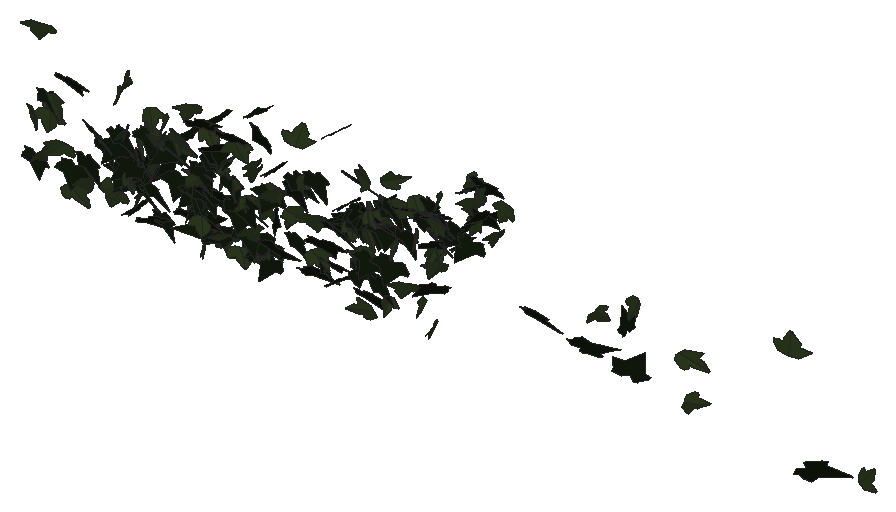
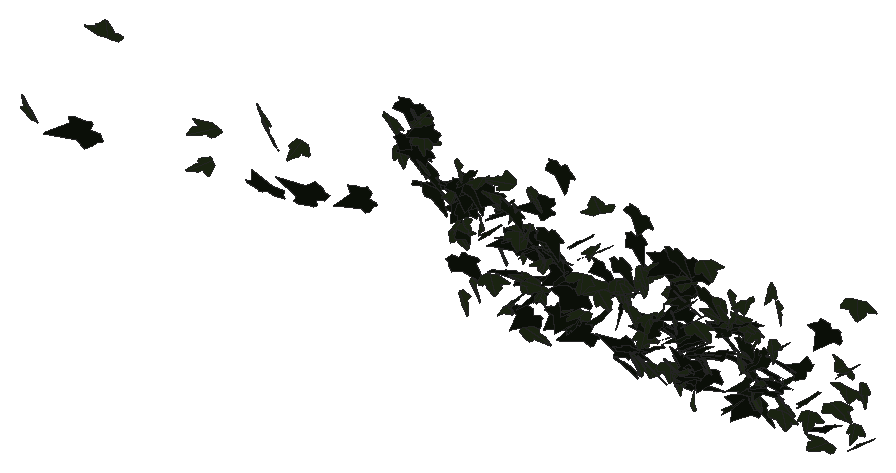
# SketchUp Ruby script. Lengths in millimetres.
U = 1.mm
M = Sketchup.active_model
def pt(a) = Geom::Point3d.new(a.map { |v| v * U })
def face(e, loops, mat)
  f = e.add_face(loops[0].map { |a| pt(a) })
  loops[1..].each { |l| e.add_face(l.map { |a| pt(a) }).erase! }
  f.material = f.back_material = mat if mat
  f
end
# faces: each face lists its corners as indices into pts; further lists are holes
def faces(e, pts, list, mat = nil) = list.each { |f| face(e, (f[0].is_a?(Array) ? f : [f]).map { |l| l.map { |i| pts[i] } }, mat) }
# xy, xz, yz: faces in a plane at the given z, y or x. An outline is a flat list of corners, or four numbers for a rectangle; further outlines are holes
def ring(l) = l.size == 4 ? [[l[0], l[1]], [l[2], l[1]], [l[2], l[3]], [l[0], l[3]]] : l.each_slice(2).to_a
def flat(e, list, mat, &to3) = list.each { |f| face(e, (f[0].is_a?(Array) ? f : [f]).map { |l| ring(l).map { |u, v| to3.(u, v) } }, mat) }
def xy(e, z, list, mat = nil) = flat(e, list, mat) { |x, y| [x, y, z] }
def xz(e, y, list, mat = nil) = flat(e, list, mat) { |x, z| [x, y, z] }
def yz(e, x, list, mat = nil) = flat(e, list, mat) { |y, z| [x, y, z] }
def lines(e, pts, list) = list.each { |a, b| e.add_line(pt(pts[a]), pt(pts[b])) }
# prism: a flat outline (further loops are holes) pulled along v
def prism(e, loops, v, mat = nil)
  f = face(e, loops, mat); d = Geom::Vector3d.new(v.map { |x| x * U })
  f.pushpull(f.normal.samedirection?(d) ? d.length : -d.length)
end
def box(e, o, s, mat = nil) = prism(e, [[o, [o[0] + s[0], o[1], o[2]], [o[0] + s[0], o[1] + s[1], o[2]], [o[0], o[1] + s[1], o[2]]]], [0, 0, s[2]], mat)
def at(x, y, z, deg = 0) = Geom::Transformation.translation(pt([x, y, z])) * Geom::Transformation.rotation(ORIGIN, Z_AXIS, deg.degrees)
def axes(o, x, y, z) = Geom::Transformation.new([*x, 0, *y, 0, *z, 0, *pt(o).to_a, 1])
def part(name) = M.definitions.add(name)
# library, detail: a bought-in or finely detailed component or shape, given as its bounding box
def library(name, o, s) = part(name).tap { |d| box(d.entities, o, s) }
def detail(e, o, s) = box(e.add_group.entities, o, s)
def put(e, d, t, mat = nil) = e.add_instance(d, t).tap { |i| i.material = mat if mat }
def group(e, t, mat = nil) = e.add_group.tap { |g| g.transformation = t; g.material = mat if mat }.entities
root = M.entities
M.materials.add("efeu1").color = [18, 25, 13]
M.materials.add("efeu2").color = [43, 57, 29]
c1 = part("ivyleaf_9")
p = [[39.1,54.8,31.7],[34.5,51.8,30.2],[-5.3,25.2,17.3],[-17.9,28.3,20.9],[-21.6,21.7,17],[-20.2,4.3,5.3],
  [-22.9,-0.3,2.5],[-17.1,-4,-0.6],[-2,-2.1,-1.2],[-0.7,-15.4,-10.1],[16.6,-22.3,-16.7],[21.1,-15.1,-12.5],
  [32.7,-10.7,-11],[46.1,-1.8,-6.6],[30.8,11.2,3.8]]
faces(c1.entities,p,[[0,1,2,3,4,5,6,7,8,9,10,11,12,13,14]],"efeu1")
c2 = part("ivyleaf_10")
p = [[0,12.8,-0.8],[-1.5,51.3,-10.9],[-4.9,51,-11.6],[-13.6,26.5,-7.3],[-13.2,15.9,-4.6],[-21.1,19.3,-7.2],
  [-29.5,16.3,-8.3],[-29.2,8.3,-6.2],[-19.7,-9.8,0.5],[-7.6,-13,4],[1,-12.2,5.8],[-0.4,51.1,-11.1],
  [-1.5,51.1,-10.9],[1,-12.4,5.9],[16.9,-12.4,3.5],[35.1,9.1,-5.1],[35,12.9,-6.1],[20.5,16.4,-4.9],
  [15.8,15,-3.8],[15.3,27.6,-7.1],[12.8,31.3,-7.8]]
faces(c2.entities,p,[[0,1,2,3,4,5,6,7,8,9,10],[11,12,0,13,14,15,16,17,18,19,20]],"efeu2")
put(root,c1,axes([3669.9,850.2,2672.9],[-0.17416,-1.02117,0.24086],[0.05118,-0.24398,-1.02417],[1.99617,-0.08284,0.04727]))
put(root,c2,axes([3698,804.6,2852.7],[1.08646,-0.66517,-0.85461],[-0.32174,0.8995,-0.81303],[2.03584,0.49713,0.32759]))
put(root,c2,axes([3702,829.9,3173.5],[-1.91435,-0.41148,0.06163],[-0.09912,-0.03545,-1.08669],[0.78563,-1.00712,0.01307]))
put(root,c2,axes([3711.1,828.5,2709.7],[-0.45389,-0.87585,-0.50942],[0.33295,0.47989,-0.90698],[1.89941,-0.29342,0.03725]))
put(root,c2,axes([3731.6,839.8,2852.3],[2.11144,-0.10197,0.14703],[0.2783,-0.01543,-1.11409],[0.19625,1.11901,-0.00197]))
put(root,c1,axes([3727.3,840.6,2921.2],[0.28219,-1.05732,0.05783],[0.00332,-0.05815,-1.06765],[2.0153,0.14814,-0.00634]))
put(root,c2,axes([3795,827.5,2761.8],[1.50681,0.45752,-0.55032],[-1.16763,0.01134,-0.87321],[-0.70132,0.96413,0.27142]))
put(root,c2,axes([3752.5,827.9,2920.7],[1.49914,-0.25929,0.7659],[1.37117,-0.26042,-0.82911],[0.69872,1.06736,-0.01623]))
put(root,c1,axes([3825.1,852.5,2684.6],[-0.7651,-0.96985,0.04167],[0.03243,-0.05214,-1.04926],[1.84724,-0.40078,0.03568]))
put(root,c1,axes([3826.2,813.7,3026.5],[1.96393,0.14353,-0.33162],[-0.64116,0.01922,-1.03998],[-0.24874,1.08372,0.06236]))
put(root,c2,axes([3834,833.2,2613.2],[1.53063,0.2367,0.68994],[1.21346,0.2707,-0.83609],[-0.67428,1.02447,0.06152]))
put(root,c2,axes([3909.3,817.4,2683.3],[-0.93066,-0.9112,-0.30006],[0.28233,0.26092,-1.03409],[1.80384,-0.51096,0.00704]))
put(root,c1,axes([3896.6,827.7,2751.1],[0.49702,-1.06639,0.03219],[0.01281,-0.03149,-1.0979],[2.03043,0.26123,-0.00095]))
put(root,c1,axes([3907.3,841.6,2857.7],[0.88542,-0.86766,0.51882],[0.44377,-0.46363,-0.98444],[1.87216,0.52025,-0.01202]))
put(root,c1,axes([3950,852.6,2817.6],[0.30365,-1.01846,0.19997],[-0.01159,-0.20323,-1.03023],[1.97532,0.15537,-0.03678]))
put(root,c2,axes([4005.9,837.7,2660.8],[-1.9519,0.1001,0.18014],[-0.38341,-0.29426,-0.98343],[-0.08266,-0.99885,0.30777]))
put(root,c2,axes([3987.3,824.9,2671.6],[1.19853,-0.51065,-0.74179],[1.10381,-0.46249,0.81075],[-1.31119,-0.85611,0.00447]))
put(root,c1,axes([4031,830.3,2846.2],[-1.86698,-0.11127,-0.32265],[0.64458,-0.19605,-0.96211],[0.08025,-1.01389,0.22145]))
put(root,c2,axes([4035,820.4,3043.2],[0.50605,-1.0177,-0.32096],[-0.02478,0.32766,-1.04972],[2.03079,0.2576,0.06717]))
put(root,c2,axes([4048.1,832.6,2902.6],[-0.09626,-1.0225,-0.34592],[0.03967,0.34531,-1.02375],[2.05399,-0.05459,0.00356]))
put(root,c1,axes([4022.3,827.8,2895.6],[0.75234,-0.92591,-0.37005],[-0.05692,0.38688,-0.99997],[1.89686,0.37885,0.11677]))
put(root,c1,axes([4061.6,835.9,2765.1],[-1.7575,-0.44266,-0.19578],[0.41975,-0.00942,-1.01897],[0.82001,-0.94392,0.10198]))
put(root,c2,axes([4062.8,818.3,3098.6],[-0.02086,-0.65902,-0.96601],[0.22835,0.96032,-0.6565],[2.21385,-0.10526,0.05862]))
put(root,c1,axes([4087.1,854.6,2731.2],[-1.76538,-0.435,0.22936],[-0.26059,-0.24184,-1.01243],[0.89891,-0.92441,0.15694]))
put(root,c1,axes([4097.6,826.9,2795],[-1.98395,-0.01938,-0.09874],[0.1908,-0.11215,-1.03642],[0.01638,-1.04107,0.11349]))
put(root,c2,axes([4081.3,814.1,2754.9],[0.35376,1.01356,0.0054],[0.0015,0.00535,-1.03046],[-1.92904,0.18588,0.00019]))
put(root,c1,axes([4083.3,825.5,2841.4],[1.72957,-0.34909,-0.4459],[-0.63884,0.34699,-0.95576],[0.86803,0.95094,0.18506]))
put(root,c2,axes([4108.4,846.9,2692],[0.40459,-0.97969,0.34164],[0.16515,-0.33073,-1.00239],[1.96775,0.22919,0.01388]))
put(root,c1,axes([4129.1,811.5,2661.6],[-0.80767,0.97747,-0.16961],[0.0991,-0.16227,-1.06549],[-1.88551,-0.42723,0.01665]))
put(root,c1,axes([4094.3,836.4,2721.9],[1.22771,-0.84105,0.05564],[0.06813,-0.04266,-1.05994],[1.60273,0.64606,0.00244]))
put(root,c1,axes([4115.8,829.1,2836.4],[1.34795,-0.38353,-0.67717],[-0.93971,0.48628,-0.79184],[1.14486,0.85071,0.14734]))
put(root,c2,axes([4120.2,817.8,2896.3],[-0.42117,0.99873,-0.22509],[0.02091,-0.22796,-1.02226],[-1.94835,-0.21834,0.03769]))
put(root,c1,axes([4153,827.4,2784.3],[-1.32671,0.647,-0.42557],[0.57818,-0.29823,-0.95102],[-1.35574,-0.76034,0.01088]))
put(root,c2,axes([4134.7,824.8,2921.7],[-1.59669,0.59742,-0.21327],[0.26377,-0.17244,-1.02824],[-1.17811,-0.84829,0.05882]))
put(root,c2,axes([4182.9,824.6,2936.6],[-0.69387,0.14567,0.98024],[-1.87868,-0.14573,-0.34549],[0.16677,-1.03564,0.18649]))
put(root,c2,axes([4156.7,846.4,2808.4],[0.14279,-1.03808,0.12585],[0.06015,-0.12387,-1.04054],[1.98922,0.07826,0.02243]))
put(root,c1,axes([4178.1,818.3,2858.8],[-0.83606,0.95911,-0.06774],[0.07245,-0.05707,-1.05487],[-1.82849,-0.4408,-0.01082]))
put(root,c1,axes([4140.3,843.7,2730.1],[1.07875,-0.86114,-0.13041],[-0.03014,0.14537,-1.02881],[1.65733,0.56316,0.06617]))
put(root,c1,axes([4176.4,845.9,2812.9],[-1.85704,-0.34148,-0.20869],[0.41497,0.00754,-1.03181],[0.63868,-0.99779,0.06362]))
put(root,c2,axes([4164.5,823.6,3016.1],[0.56951,1.09198,-0.17073],[-0.11915,-0.15984,-1.1321],[-2.10014,0.30519,0.01793]))
put(root,c2,axes([4168.5,843.2,2811.6],[0.15033,-0.95431,0.43372],[0.34481,-0.41598,-0.94826],[1.965,0.146,0.13322]))
put(root,c1,axes([4172.3,830.6,2932.7],[-0.9679,-0.94321,-0.09432],[0.05731,0.0909,-1.07145],[1.80315,-0.50918,-0.01657]))
put(root,c1,axes([4167.8,806.6,2633.6],[1.50685,0.67685,0.12793],[0.18914,0.08063,-1.04162],[-1.29727,0.79795,-0.00327]))
put(root,c2,axes([4216.9,814,2927.6],[0.00117,0.13162,1.05151],[-0.66028,0.99359,-0.12416],[-1.9057,-0.34418,0.04367]))
put(root,c1,axes([4191.7,850.7,2632.8],[0.43653,-1.0033,0.0634],[-0.00129,-0.06518,-1.02908],[1.9133,0.22886,-0.01516]))
put(root,c2,axes([4227,822.5,3010.4],[0.64338,-1.0447,-0.00092],[0.01246,0.00309,-1.09801],[1.98823,0.33804,0.00718]))
put(root,c1,axes([4245.4,831.4,2865.2],[-1.54309,0.45568,-0.52869],[0.81465,-0.31545,-0.92833],[-1.04923,-0.91508,0.05675]))
put(root,c1,axes([4257.9,833.9,2903.9],[-1.79694,-0.47383,0.23394],[-0.4188,-0.08294,-1.05612],[0.91437,-0.96918,-0.02399]))
put(root,c1,axes([4215.5,842.9,2901.1],[0.74292,-0.86605,0.48781],[0.78845,-0.33463,-0.92562],[1.7196,0.52759,0.21365]))
put(root,c1,axes([4269.6,847.4,2801.7],[-1.03337,-0.90726,0.00395],[-0.00347,-0.00351,-1.05732],[1.72671,-0.54297,0.00024]))
put(root,c2,axes([4278.6,820.6,2970.8],[-1.64011,0.59298,0.20748],[-0.33821,0.10774,-1.04601],[-1.14683,-0.87982,0.01175]))
put(root,c2,axes([4244.5,840.7,2927.8],[0.12335,0.0127,1.18772],[2.24987,-0.11645,-0.06326],[0.22,1.18378,-0.01897]))
put(root,c1,axes([4334.6,831.2,2996.4],[-0.87454,0.96714,0.04112],[-0.04025,0.03548,-1.07075],[-1.84189,-0.45998,0.00387]))
put(root,c2,axes([4330.7,823.2,3093.5],[-1.14244,-0.87702,0.25844],[-0.11213,-0.27142,-1.0579],[1.7365,-0.59452,0.10172]))
put(root,c2,axes([4318.2,835.9,2745.1],[1.00135,-0.83541,0.33377],[0.48748,-0.23155,-0.98332],[1.64129,0.57846,0.08842]))
put(root,c1,axes([4337.5,853.1,2770.8],[-1.42849,-0.65112,0.33645],[-0.2605,-0.34857,-0.97993],[1.37032,-0.74502,0.16444]))
put(root,c1,axes([4321.9,822,2706],[1.55032,0.65168,-0.14431],[-0.2017,-0.09852,-1.04313],[-1.2542,0.82138,-0.01063]))
put(root,c2,axes([4373.2,824,2851.9],[-1.51746,-0.32726,0.62113],[-0.85896,-0.48102,-0.83279],[1.0235,-0.8889,0.22198]))
put(root,c1,axes([4365.1,828.3,2752.5],[-1.41251,0.35638,-0.65274],[1.00684,-0.39515,-0.81725],[-0.99479,-0.90596,0.09968]))
put(root,c1,axes([4354.6,844.3,2777.7],[-0.62927,-0.97685,0.19643],[-0.18843,-0.17372,-1.03061],[1.88697,-0.34311,-0.03741]))
put(root,c1,axes([4399.2,848.8,2648.1],[-1.46775,-0.11484,0.84238],[-1.57813,-0.14946,-0.77951],[0.35718,-1.13226,0.01746]))
put(root,c1,axes([4365.4,843.1,2783.7],[-0.4246,-1.0258,0.17771],[-0.02906,-0.1785,-1.04953],[1.98117,-0.22246,0.02269]))
put(root,c2,axes([4369.5,829.2,2689.7],[1.29866,0.80377,-0.07318],[-0.10086,-0.05101,-1.05432],[-1.53274,0.68437,0.00737]))
put(root,c2,axes([4362.5,848.8,2586.1],[0.1001,-0.06848,1.13998],[1.21539,-0.94434,-0.08619],[1.80196,0.64075,-0.00519]))
put(root,c1,axes([4365.9,832.2,2880.5],[0.18721,-1.07427,-0.09221],[-0.00741,0.09224,-1.07876],[2.05206,0.09834,0.00451]))
put(root,c1,axes([4363.5,808,3058.7],[1.9174,0.44244,0.15073],[0.26893,0.05309,-1.1003],[-0.84796,1.01729,-0.00813]))
put(root,c1,axes([4352.4,850.4,2685.7],[0.48432,-0.52196,1.01173],[0.95764,-0.87837,-0.57972],[1.94355,0.56287,0.03353]))
put(root,c1,axes([4374.1,843.6,2794.6],[-0.04482,-1.03029,-0.27005],[-0.00316,0.27015,-1.03053],[2.02708,-0.02236,-0.00758]))
put(root,c1,axes([4363.2,841.3,2694.5],[-0.10504,-0.06408,1.06097],[1.40093,-0.76871,-0.00814],[1.45931,0.73335,0.08418]))
put(root,c2,axes([4395.8,832.6,3021.4],[1.09062,0.89184,0.18458],[0.16171,0.16478,-1.05994],[-1.72577,0.57905,0.01733]))
put(root,c1,axes([4410.4,813.4,2817.5],[1.73249,0.44583,-0.40687],[-0.66916,-0.20676,-1.01321],[-0.9337,0.97542,-0.0288]))
put(root,c1,axes([4397.8,834.9,2925.5],[0.84187,-0.90867,-0.3788],[0.00024,0.41533,-0.99616],[1.87363,0.40823,0.17033]))
put(root,c1,axes([4396.3,830.2,2946],[1.17813,-0.89247,-0.02327],[0.1527,0.08382,-1.08017],[1.69225,0.61377,0.11367]))
put(root,c1,axes([4402.1,829.4,2906.2],[2.01072,-0.2578,-0.00147],[0.00427,0.01542,-1.08738],[0.49064,1.05638,0.01551]))
put(root,c1,axes([4453,828.8,3098.3],[-0.66563,1.02892,-0.0112],[-0.04779,-0.02036,-1.08631],[-1.95777,-0.34933,0.03033]))
put(root,c1,axes([4406.2,824.5,2809],[1.24895,-0.76037,-0.3642],[-0.11255,0.41887,-0.98107],[1.60062,0.62276,0.2152]))
put(root,c1,axes([4422.8,804.5,2987.1],[1.21972,0.75897,0.40754],[0.44216,0.33686,-0.99267],[-1.5788,0.68069,0.03685]))
put(root,c1,axes([4463.1,824.9,2949.7],[-1.81031,0.53547,0.04189],[-0.07388,0.01643,-1.09155],[-1.01955,-0.95197,0.00472]))
put(root,c2,axes([4442.9,835.3,2646.9],[1.41868,-0.61204,-0.39838],[-0.23898,0.45337,-0.93147],[1.36917,0.71331,0.25021]))
put(root,c2,axes([4453,838,2870.4],[0.75404,-0.96529,-0.257],[-0.01266,0.27392,-1.0391],[1.90109,0.38469,0.09501]))
put(root,c1,axes([4484.3,820.7,2674.3],[-1.51842,0.64432,0.02333],[-0.10656,-0.03226,-1.02374],[-1.22244,-0.79751,0.06026]))
put(root,c2,axes([4477.7,821.8,2668.1],[-1.39467,-0.71537,-0.04037],[0.07193,0.01907,-1.02401],[1.36177,-0.73367,0.01274]))
put(root,c2,axes([4475.6,800.2,2930.5],[0.24157,-0.46512,1.05499],[-0.33937,1.04067,0.48026],[-2.16793,-0.21474,0.04237]))
put(root,c1,axes([4477,843.6,2871.7],[0.28825,-1.05206,0.06443],[0.0115,-0.06422,-1.0629],[2.006,0.15154,-0.00316]))
put(root,c1,axes([4480,815.2,3048.2],[2.06916,0.15846,-0.03375],[-0.07278,0.02847,-1.09817],[-0.29963,1.08735,0.03367]))
put(root,c2,axes([4506,827.9,2867.4],[-0.17968,0.97241,-0.40538],[-0.08339,-0.41028,-0.97395],[-2.00333,-0.07014,0.0769]))
put(root,c1,axes([4514.1,847.5,2758],[-0.60949,-0.94857,0.31634],[0.02002,-0.33535,-0.99491],[1.90296,-0.30029,0.11179]))
put(root,c2,axes([4519.8,822.6,3017.8],[-1.33014,-0.79219,-0.30752],[0.84674,-0.00187,-1.0063],[1.37794,-0.76356,0.32152]))
put(root,c2,axes([4545.6,838.2,2805.5],[-0.33284,-1.04729,0.05785],[0.37063,-0.09005,-1.0415],[1.96154,-0.16069,0.20661]))
put(root,c1,axes([4517.2,843.2,2801.3],[1.40006,-0.65,0.38792],[0.53049,-0.27032,-0.98152],[1.33941,0.78649,-0.01675]))
put(root,c1,axes([4528.8,823.8,2817.6],[-0.8672,-0.41074,-0.91799],[1.55562,0.43592,-0.60076],[1.11515,-0.92752,0.12417]))
put(root,c2,axes([4539.3,816.2,2640.4],[1.69923,0.43868,0.24577],[0.44332,0.08302,-0.9944],[-0.84812,0.92231,-0.02738]))
put(root,c1,axes([4582.6,828.7,2653],[-1.60207,0.56961,-0.05662],[0.09258,-0.02914,-1.01639],[-1.08549,-0.84318,-0.00312]))
put(root,c2,axes([4555.4,830.1,2827.2],[0.55785,1.02348,0.03769],[-0.11655,0.05665,-1.06202],[-1.94572,0.29004,0.07442]))
put(root,c1,axes([4557.1,832.1,2710.3],[-0.34319,-1.0131,-0.20221],[0.13937,0.19222,-1.02834],[1.96123,-0.19094,0.03769]))
put(root,c2,axes([4593.3,831,2952.4],[-0.33928,-1.06893,-0.03979],[-0.0385,0.0437,-1.08336],[2.03544,-0.17735,-0.02713]))
put(root,c2,axes([4593.8,825.1,2981],[-0.30344,-1.08106,0.02862],[0.00559,-0.02937,-1.09273],[2.05819,-0.1593,0.00719]))
put(root,c2,axes([4590.9,813.9,2737.8],[-0.91247,-0.90072,-0.37557],[0.38233,0.31839,-1.02004],[1.81752,-0.51917,0.02602]))
put(root,c1,axes([4619.9,822.4,3092.9],[0.87127,0.08634,-1.10755],[-2.10184,0.16518,-0.4436],[0.22912,1.187,0.14229]))
put(root,c1,axes([4607.5,811.1,3174.4],[0.56002,0.92645,0.52974],[-0.05912,0.55671,-0.95636],[-2.03025,0.23934,0.17397]))
put(root,c2,axes([4600.6,844.3,2657.3],[1.43932,-0.72269,0.01223],[-0.00551,-0.02073,-1.04591],[1.37561,0.75608,-0.01699]))
put(root,c2,axes([4612.2,843.2,2665.1],[1.54057,-0.66459,0.01205],[0.01534,-0.00917,-1.04734],[1.26497,0.8095,-0.00197]))
put(root,c1,axes([4643,850.9,2687.6],[-1.7581,-0.37392,0.24336],[-0.43404,-0.08518,-0.99654],[0.72977,-0.95147,-0.00642]))
put(root,c2,axes([4633,830.6,2829],[1.63471,-0.58825,-0.24217],[-0.17832,0.28548,-1.02575],[1.19752,0.84552,0.17785]))
put(root,c1,axes([4651.9,844.5,2628.3],[-1.77465,0.00042,-0.43465],[0.82072,-0.12795,-0.92524],[-0.1036,-1.0208,0.11579]))
put(root,c1,axes([4654.7,839.1,2879],[-1.18018,-0.82302,0.29027],[0.02945,-0.3664,-1.00581],[1.66067,-0.57839,0.22412]))
put(root,c1,axes([4676.9,833.5,2985.3],[-0.63203,1.01356,-0.1565],[0.05172,-0.15574,-1.06634],[-1.95117,-0.33244,0.02243]))
put(root,c2,axes([4666,832.4,2900.2],[1.53874,-0.67201,-0.18203],[-0.22898,0.1399,-1.05088],[1.30512,0.81685,0.03024]))
put(root,c2,axes([4667.7,818.6,2901.9],[-0.74413,-0.992,-0.26862],[0.18649,0.25011,-1.06627],[1.94706,-0.40308,-0.00053]))
put(root,c1,axes([4637.9,840.1,2674.4],[0.69436,-0.29991,0.91578],[1.4261,-0.52741,-0.47124],[1.15316,0.83283,0.03135]))
put(root,c1,axes([4689.9,806,2817.6],[0.48459,-0.22787,-1.11533],[-1.61743,0.72234,-0.34159],[1.44146,0.88713,-0.00834]))
put(root,c2,axes([4688.9,827.8,2900.2],[-0.76854,-0.99757,-0.03403],[-0.00695,0.03818,-1.07606],[1.89967,-0.40344,-0.0177]))
put(root,c2,axes([4749.6,836.6,2838.9],[-0.55176,-0.98191,0.31894],[-0.08655,-0.31881,-1.02284],[1.96297,-0.29006,0.04455]))
put(root,c1,axes([4737.2,837.7,2942.1],[-0.51716,-0.01761,-1.03792],[1.97531,0.01554,-0.27199],[0.03711,-1.07279,0.01309]))
put(root,c1,axes([4747.5,831.3,2757.9],[0.80289,-0.94909,-0.08441],[-0.0612,0.07808,-1.03862],[1.8124,0.42308,0.00232]))
put(root,c2,axes([4749.5,813,2855.6],[0.63511,0.3441,0.95667],[0.90244,0.838,-0.46681],[-1.7116,0.56952,0.10886]))
put(root,c2,axes([4776.1,809.2,3132.3],[1.40816,0.84599,-0.48301],[0.62082,0.35637,1.12384],[1.747,-0.80854,-0.01004]))
put(root,c1,axes([4764.8,816.8,2991.6],[0.76785,-0.89232,-0.45673],[0.05161,0.50187,-0.95656],[1.9071,0.34569,0.20978]))
put(root,c2,axes([4795.6,816.3,2990.5],[0.28172,1.07471,0.00521],[-0.01094,0.00605,-1.08483],[-2.04538,0.14799,0.00652]))
put(root,c2,axes([4841.7,822.5,2865.9],[-1.84788,-0.47407,-0.06035],[0.09767,0.03245,-1.08047],[0.90427,-0.97227,-0.00663]))
put(root,c1,axes([4818.6,815.9,2670.4],[1.8857,0.19349,0.34196],[0.63533,0.07469,-1.00948],[-0.39437,1.04549,0.00883]))
put(root,c1,axes([4833.7,831.3,3011.3],[0.21764,-1.05858,-0.20086],[-0.06451,0.19836,-1.06467],[2.04962,0.11865,-0.01218]))
put(root,c2,axes([4843.2,820.9,2732.2],[1.05487,0.87957,0.5498],[0.43341,0.50497,-1.03743],[-1.92596,0.59539,0.06767]))
put(root,c1,axes([4859,853.9,2685],[-0.23484,-0.38649,0.96478],[-0.21097,-0.96112,-0.3992],[1.96674,-0.14925,0.07238]))
put(root,c1,axes([4871.8,814.1,2792.8],[2.01018,0.4368,-0.28002],[-0.49276,-0.10666,-1.14297],[-0.85574,1.08748,0.00037]))
put(root,c1,axes([4894.4,827.2,2720],[1.76017,0.35972,-0.30435],[-0.6915,0.11756,-0.96516],[-0.57099,0.96651,0.23066]))
put(root,c1,axes([4891.4,826,2861.9],[1.99652,0.08714,0.11459],[0.22065,-0.0117,-1.05244],[-0.16243,1.05521,-0.02114]))
put(root,c1,axes([4945,803.2,3229.1],[0.11547,1.11423,0.15178],[0.01043,0.1517,-1.11587],[-2.14015,0.06086,0.00275]))
put(root,c1,axes([4912,835.3,2854.4],[1.3333,-0.78526,0.03083],[0.11312,0.01176,-1.05105],[1.49138,0.70114,0.05216]))
put(root,c1,axes([4939.8,798.2,2674.1],[0.90438,0.66369,0.75251],[0.62468,0.684,-0.81053],[-1.80455,0.5694,0.09655]))
put(root,c1,axes([4975.1,809.6,2919.9],[-0.32512,1.00321,0.31999],[-0.2836,0.29788,-1.01344],[-1.98392,-0.20698,0.09243]))
put(root,c1,axes([4984.3,811.7,2973.9],[-0.08673,1.09241,-0.10476],[0.05246,-0.10368,-1.09312],[-2.08796,-0.04798,-0.02311]))
put(root,c2,axes([4979.8,835.2,2883.5],[0.85835,0.94161,-0.02503],[-0.02651,-0.02108,-1.04404],[-1.7925,0.4512,0.00346]))
put(root,c1,axes([5024,841,2903.9],[-0.40512,-0.32121,-0.99616],[-1.05775,-0.82672,0.38533],[-1.68799,0.59514,-0.00238]))
put(root,c1,axes([5017,819.9,2953.6],[-1.41495,0.73663,-0.22142],[0.1562,-0.23021,-1.04146],[-1.45555,-0.74078,0.10347]))
put(root,c2,axes([4992.3,845.4,2769.6],[-0.17477,0.939,-0.42122],[0.02437,-0.42182,-0.94312],[-1.95852,-0.08904,0.02585]))
put(root,c2,axes([5035.2,837.4,2774.8],[-1.70008,-0.10422,0.56888],[-1.02747,-0.2252,-0.88896],[0.39482,-1.03482,0.13617]))
put(root,c2,axes([4995.9,843.5,2885.6],[-0.26298,0.15546,-1.04467],[0.88971,-0.93575,-0.20109],[-1.80249,-0.48457,0.05316]))
put(root,c1,axes([4981.7,819.5,3073.9],[1.73029,-0.54833,0.2968],[0.63305,-0.01732,-1.05089],[1.00369,0.95621,0.15116]))
put(root,c1,axes([5010.7,839.6,2923.6],[-0.36118,-1.04973,-0.09161],[0.017,0.09148,-1.06672],[2.00537,-0.18984,-0.00745]))
put(root,c2,axes([5060,826.5,2598.6],[-0.75744,0.03149,0.95846],[-1.78066,-0.24041,-0.3806],[0.40041,-1.00957,0.12053]))
put(root,c1,axes([5016.6,809.9,2742.1],[0.83868,-0.05563,-1.07306],[-0.83677,1.04893,-0.23493],[1.86596,0.49538,0.37695]))
put(root,c1,axes([5062.6,813.7,2931.8],[-0.52734,0.87515,0.55939],[-0.46507,0.50778,-0.91544],[-1.92129,-0.36312,0.06806]))
put(root,c2,axes([5061.7,807.3,3090.3],[0.29235,-0.32446,-1.20122],[-1.10832,1.05085,-0.35831],[2.09272,0.60186,-0.02196]))
put(root,c2,axes([5050.5,836.2,2974.1],[-0.28713,0.95695,-0.45403],[0.02933,-0.45658,-0.96745],[-2.01565,-0.14296,0.0506]))
put(root,c2,axes([5023.2,844.2,2791.7],[-0.37857,0.09621,-1.0405],[1.86757,-0.34687,-0.21966],[-0.68357,-1.00095,-0.02389]))
put(root,c1,axes([5032.9,842.8,2936.1],[0.15861,-0.2082,1.04216],[0.71923,-0.97123,-0.22425],[1.89043,0.38698,-0.00212]))
put(root,c1,axes([5064.3,837.2,2785.4],[-0.92962,-0.86812,0.31716],[-0.36369,-0.25611,-0.99533],[1.721,-0.52305,-0.03902]))
put(root,c1,axes([5046.1,824.3,2659.4],[2.00418,0.05494,-0.12972],[-0.2465,-0.00719,-1.05449],[-0.10546,1.06099,-0.00043]))
put(root,c2,axes([5061.5,821.2,2887.1],[-0.09712,1.0448,0.0032],[0.00658,0.00337,-1.04604],[-1.98847,-0.05102,-0.00362]))
put(root,c2,axes([5087.9,839.8,2941.6],[-1.78435,-0.4727,0.04378],[-0.06113,-0.03353,-1.04987],[0.90143,-0.93798,0.01546]))
put(root,c2,axes([5085,815.4,2965.9],[1.01565,0.91545,0.1932],[0.08966,0.19584,-1.05811],[-1.77841,0.53269,0.05699]))
put(root,c1,axes([5085.5,837.3,2714.9],[0.7423,-0.9262,-0.29678],[-0.18866,0.28023,-1.00483],[1.84139,0.40208,0.01669]))
put(root,c1,axes([5103,833.2,2924.2],[-0.72619,-0.98328,-0.03529],[0.01944,0.03389,-1.05471],[1.87248,-0.38169,-0.00274]))
put(root,c1,axes([5136.7,817.5,3021.4],[-0.25884,1.02686,0.32023],[-0.27846,0.30212,-1.03092],[-2.02812,-0.17253,0.10067]))
put(root,c2,axes([5117.1,824.9,3019.5],[-0.85892,0.99422,-0.05253],[-0.00073,-0.05785,-1.09158],[-1.89483,-0.45065,0.02423]))
put(root,c1,axes([5085.4,833,2915.9],[1.9178,-0.24895,0.30361],[0.56882,-0.05592,-1.03783],[0.48456,1.05093,0.01669]))
put(root,c1,axes([5125,834.3,2923.5],[-0.92989,-0.93303,-0.00792],[0.38576,-0.09741,-1.02896],[1.7334,-0.47885,0.22474]))
put(root,c2,axes([5137.8,833.2,2661],[0.45206,0.84721,-0.56766],[-0.26917,-0.54986,-0.87982],[-1.92215,0.27625,-0.0103]))
put(root,c1,axes([5146.7,846.8,2794.5],[-1.36058,-0.78039,-0.02428],[0.24255,-0.08416,-1.04754],[1.46603,-0.71034,0.15078]))
put(root,c2,axes([5153.2,847,2866.5],[0.99734,-0.88255,0.26397],[0.28314,-0.21863,-1.02628],[1.73017,0.54451,0.01578]))
put(root,c2,axes([5144.8,819.6,3108.3],[-0.18152,-0.31554,1.0512],[0.65667,0.99305,0.32938],[-1.98293,0.35774,0.01285]))
put(root,c1,axes([5139.4,836.3,3010.2],[0.36508,-0.93138,-0.50614],[0.24796,0.53118,-0.92807],[2.00213,0.10405,0.20723]))
put(root,c1,axes([5153,832.8,3018.6],[0.3149,-1.04814,0.20582],[0.00167,-0.20814,-1.06066],[2.03291,0.16253,-0.03101]))
put(root,c2,axes([5208,833.1,2739.9],[-1.42863,-0.73163,0.14522],[-0.16512,-0.11898,-1.04793],[1.40996,-0.75525,0.02442]))
put(root,c2,axes([5209.5,822.7,3037],[1.91165,-0.14869,-0.34824],[-0.63431,0.12137,-1.01315],[0.34204,1.05614,0.0674]))
put(root,c1,axes([5193.3,848,2922.4],[0.31562,-1.03842,0.11729],[0.03466,-0.11587,-1.05158],[1.98859,0.16683,-0.00029]))
put(root,c1,axes([5221.1,805.1,3040.4],[1.78103,0.53696,0.15029],[-0.00909,0.30131,-1.04682],[-1.06117,0.89863,0.2612]))
put(root,c2,axes([5241.9,844.5,2939.9],[-0.59332,0.83029,-0.58184],[-0.20716,-0.63262,-0.84442],[-1.91842,-0.18847,0.27113]))
put(root,c1,axes([5279.1,822.4,3036.7],[0.0355,1.05808,0.18125],[-0.1353,0.1821,-1.0557],[-2.03858,0.00634,0.07323]))
put(root,c2,axes([5259.7,815.8,3080],[0.58399,1.0429,0.11688],[0.09526,0.10709,-1.08696],[-1.995,0.3104,-0.01769]))
put(root,c2,axes([5274.4,839.1,2694.3],[0.84711,-0.99315,0.0222],[0.01389,-0.02105,-1.08832],[1.89058,0.44515,-0.00195]))
put(root,c1,axes([5281.8,806.9,3038.5],[1.20556,-0.49743,-0.7037],[-0.55046,0.69998,-0.75515],[1.54496,0.63755,0.28005]))
put(root,c1,axes([5325.9,840.3,2774.2],[-0.04106,0.70195,-0.80631],[-0.42548,-0.7916,-0.68317],[-1.98963,0.1548,0.16274]))
put(root,c1,axes([5316.1,821.9,3036],[0.90626,0.98201,-0.12024],[-0.11117,-0.10531,-1.09135],[-1.87963,0.4797,0.00657]))
put(root,c2,axes([5318.5,836.1,2902.8],[0.40503,0.8897,-0.56607],[-0.51498,-0.51207,-0.90656],[-1.93976,0.32172,0.12248]))
put(root,c2,axes([5325.5,832.2,2633.1],[0.301,-1.1246,-0.12054],[-0.03107,0.11943,-1.13567],[2.15238,0.15899,0.00046]))
put(root,c2,axes([5339.8,817,3026.1],[1.62306,-0.23315,-0.60781],[-0.98902,0.35952,-0.86704],[0.74623,0.98359,0.17284]))
put(root,c1,axes([5298.7,834.9,3079.1],[0.98337,-0.94339,-0.08218],[0.05309,0.10874,-1.0729],[1.80148,0.51176,0.07648]))
put(root,c1,axes([5327.5,817.6,2870.3],[0.38871,0.45591,0.94787],[0.44595,0.92159,-0.49376],[-1.9515,0.30141,0.07597]))
put(root,c1,axes([5297.2,842.2,2965.7],[1.16165,-0.78535,0.386],[0.4241,-0.31562,-0.99451],[1.61056,0.64956,-0.01653]))
put(root,c2,axes([5343.9,831.5,2860.9],[-0.95386,-0.88341,0.35046],[-0.30937,-0.31069,-1.01561],[1.78212,-0.52677,0.01128]))
put(root,c2,axes([5345.5,832.6,3109.3],[0.54556,-1.02814,-0.17905],[0.00053,0.18576,-1.06621],[1.98622,0.28235,0.04947]))
put(root,c1,axes([5334.8,799,2954.2],[1.21095,0.80949,0.29164],[0.33022,0.23455,-1.02959],[-1.60392,0.65945,0.00821]))
put(root,c2,axes([5339.4,835.2,2910],[-0.22593,1.02572,-0.30688],[-0.0115,-0.3094,-1.0318],[-2.03762,-0.11198,0.03985]))
put(root,c1,axes([5313.3,831.3,3041.4],[1.22696,-0.78764,0.37214],[0.4667,-0.28016,-1.01777],[1.59089,0.68965,0.01156]))
put(root,c2,axes([5354,834.4,3007.6],[0.44324,1.05288,-0.03205],[0.01448,-0.03451,-1.07822],[-2.00471,0.23254,-0.01487]))
put(root,c1,axes([5426.1,814.5,3003.2],[-1.26439,0.55926,0.64391],[-0.96146,0.39957,-0.86826],[-1.30779,-0.83446,0.01579]))
put(root,c1,axes([5455.6,827.6,2983.9],[-0.5266,1.04891,-0.09655],[-0.00016,-0.09984,-1.08449],[-2.00473,-0.27552,0.02544]))
put(root,c1,axes([5476.5,825.3,3053.8],[-0.68628,1.02452,0.01335],[0.00038,0.01423,-1.08611],[-1.95003,-0.36056,-0.00491]))
put(root,c1,axes([5477.8,831.7,2995.7],[-1.66365,-0.64284,0.00344],[0.0652,-0.05239,-1.08326],[1.22174,-0.87257,0.0625]))
put(root,c1,axes([5467.7,814.1,3191.9],[1.13172,0.48775,0.77032],[0.8049,0.66719,-0.74892],[-1.53728,0.70841,0.17497]))
put(root,c2,axes([5490.6,825.3,3153.6],[-1.15818,-0.90255,-0.02439],[0.08986,-0.00243,-1.08779],[1.71601,-0.60903,0.0405]))
put(root,c2,axes([5490.2,844.6,3072],[1.41741,-0.77737,0.06495],[0.07025,-0.05458,-1.07649],[1.48297,0.74558,-0.01108]))
put(root,c2,axes([5484.3,813,3230.8],[-0.1795,-0.48221,-0.99741],[0.85032,0.89945,-0.4771],[1.92942,-0.44126,0.11747]))
put(root,c1,axes([5520.5,828.8,3113.3],[1.27845,0.36495,-0.77532],[-1.3289,-0.33798,-0.76404],[-0.94542,0.96857,0.02553]))
put(root,c2,axes([5520.8,814.7,3191.4],[-0.04669,0.70818,0.84605],[-0.52385,0.81557,-0.69065],[-2.03344,-0.22636,0.1585]))
put(root,c2,axes([5533.1,818.5,3226.1],[0.8911,-0.9192,-0.36578],[-0.32242,0.3242,-1.03157],[1.85503,0.49791,-0.00359]))
put(root,c1,axes([5559.1,820.7,3134.7],[-0.27799,0.78644,-0.75317],[-0.22539,-0.76688,-0.77779],[-2.06015,-0.02222,0.18673]))
put(root,c1,axes([5546.7,807.9,3247.2],[1.56224,0.31762,-0.69178],[-1.28827,-0.16081,-0.87703],[-0.6627,1.06136,0.07414]))
put(root,c2,axes([5595.3,818.7,3071.8],[-0.42955,-1.07935,0.00265],[-0.0084,-0.00179,-1.10269],[2.05421,-0.22571,-0.00395]))
put(root,c2,axes([5628.7,822.1,3176.4],[1.70388,-0.61628,-0.14478],[-0.153,0.13807,-1.08478],[1.19509,0.89633,0.06755]))
put(root,c1,axes([5735.9,811.2,2840.1],[2.0983,-0.21918,0.19676],[0.37158,-0.02693,-1.12403],[0.4197,1.1196,0.01148]))
put(root,c1,axes([5943,824.9,2774],[0.33508,-0.22665,1.11858],[2.11212,-0.23021,-0.22132],[0.50706,1.1087,0.18271]))
put(root,c2,axes([6016,806.2,2936.8],[-0.64974,-0.77327,-0.80365],[0.76454,0.69878,-0.84302],[1.98008,-0.52355,0.06179]))
put(root,c1,axes([6146.9,797.6,2925.9],[0.03716,0.46169,1.12863],[-0.21895,1.12444,-0.45798],[-2.31043,-0.09913,0.06155]))
put(root,c1,axes([6132.8,830.1,2739.9],[-1.56373,0.38612,0.72618],[1.25518,-0.30397,0.90783],[0.93523,1.05357,-0.00422]))
put(root,c2,axes([6161.3,822.3,3011.7],[1.39857,-1.01341,0.00235],[0.0025,-0.00194,-1.2518],[1.92872,0.73485,-0.00008]))
put(root,c2,axes([6363.7,827.2,2885.3],[0.92186,0.52661,0.95369],[1.24297,0.69501,-0.71547],[-1.65951,0.81309,-0.00611]))
put(root,c2,axes([6393.9,808.1,2738.6],[-0.26299,-0.37024,-1.1162],[1.25817,0.90503,-0.38204],[1.85105,-0.66776,0.10109]))
put(root,c2,axes([6805.6,813.4,3070.1],[2.32629,0.15922,-0.02687],[0.04652,0.02037,1.23251],[0.30378,-1.22243,0.01703]))
put(root,c1,axes([6897.1,795,2677],[0.37182,0.41996,-1.27558],[0.58049,1.24145,0.45544],[2.48908,-0.35226,0.08433]))
put(root,c2,axes([7092.2,837.3,2678.3],[1.56416,-0.8309,-0.44817],[0.60187,-0.31757,1.16869],[-1.69294,-0.8806,0.00142]))
